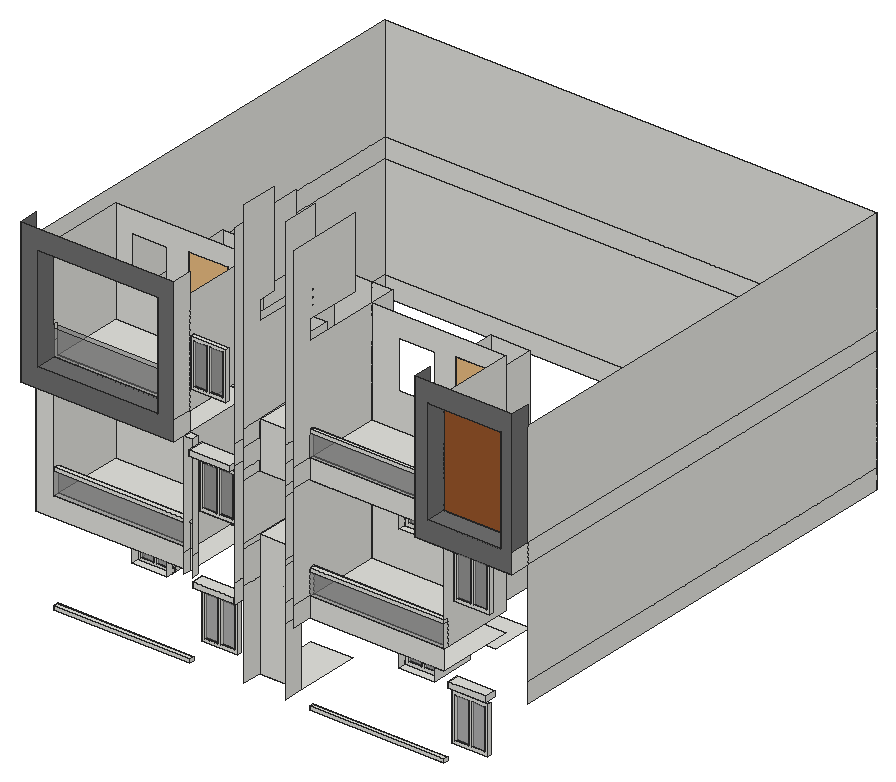
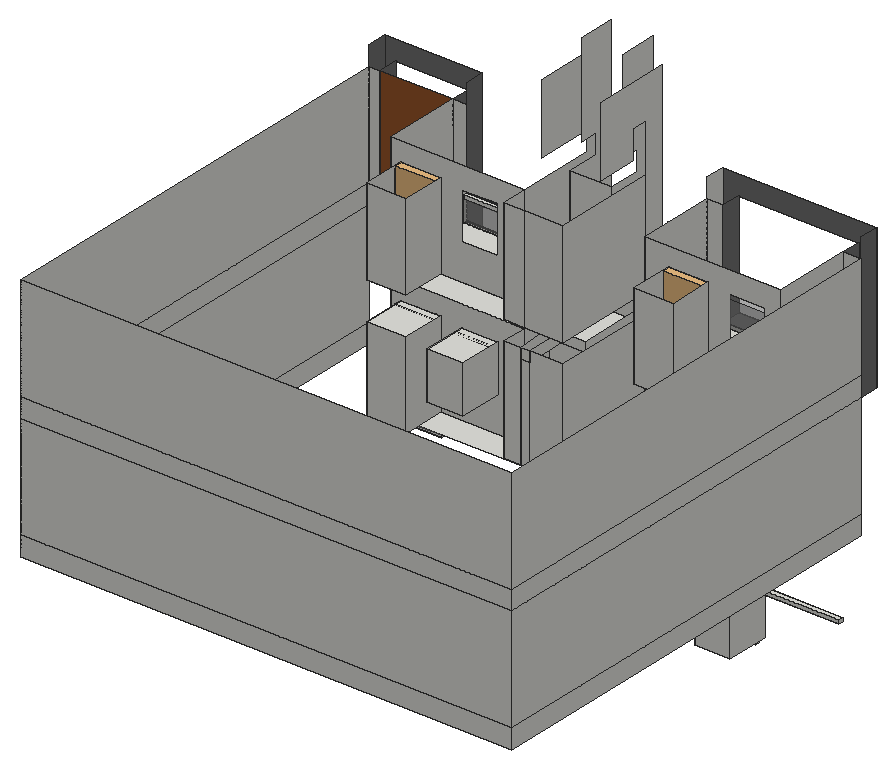
# SketchUp Ruby script. Lengths in inches.
U = 1.inch
M = Sketchup.active_model
def pt(a) = Geom::Point3d.new(a.map { |v| v * U })
def face(e, loops, mat)
  f = e.add_face(loops[0].map { |a| pt(a) })
  loops[1..].each { |l| e.add_face(l.map { |a| pt(a) }).erase! }
  f.material = f.back_material = mat if mat
  f
end
# faces: each face lists its corners as indices into pts; further lists are holes
def faces(e, pts, list, mat = nil) = list.each { |f| face(e, (f[0].is_a?(Array) ? f : [f]).map { |l| l.map { |i| pts[i] } }, mat) }
# xy, xz, yz: faces in a plane at the given z, y or x. An outline is a flat list of corners, or four numbers for a rectangle; further outlines are holes
def ring(l) = l.size == 4 ? [[l[0], l[1]], [l[2], l[1]], [l[2], l[3]], [l[0], l[3]]] : l.each_slice(2).to_a
def flat(e, list, mat, &to3) = list.each { |f| face(e, (f[0].is_a?(Array) ? f : [f]).map { |l| ring(l).map { |u, v| to3.(u, v) } }, mat) }
def xy(e, z, list, mat = nil) = flat(e, list, mat) { |x, y| [x, y, z] }
def xz(e, y, list, mat = nil) = flat(e, list, mat) { |x, z| [x, y, z] }
def yz(e, x, list, mat = nil) = flat(e, list, mat) { |y, z| [x, y, z] }
def lines(e, pts, list) = list.each { |a, b| e.add_line(pt(pts[a]), pt(pts[b])) }
# prism: a flat outline (further loops are holes) pulled along v
def prism(e, loops, v, mat = nil)
  f = face(e, loops, mat); d = Geom::Vector3d.new(v.map { |x| x * U })
  f.pushpull(f.normal.samedirection?(d) ? d.length : -d.length)
end
def box(e, o, s, mat = nil) = prism(e, [[o, [o[0] + s[0], o[1], o[2]], [o[0] + s[0], o[1] + s[1], o[2]], [o[0], o[1] + s[1], o[2]]]], [0, 0, s[2]], mat)
def at(x, y, z, deg = 0) = Geom::Transformation.translation(pt([x, y, z])) * Geom::Transformation.rotation(ORIGIN, Z_AXIS, deg.degrees)
def axes(o, x, y, z) = Geom::Transformation.new([*x, 0, *y, 0, *z, 0, *pt(o).to_a, 1])
def part(name) = M.definitions.add(name)
# library, detail: a bought-in or finely detailed component or shape, given as its bounding box
def library(name, o, s) = part(name).tap { |d| box(d.entities, o, s) }
def detail(e, o, s) = box(e.add_group.entities, o, s)
def put(e, d, t, mat = nil) = e.add_instance(d, t).tap { |i| i.material = mat if mat }
def group(e, t, mat = nil) = e.add_group.tap { |g| g.transformation = t; g.material = mat if mat }.entities
root = M.entities
M.materials.add("Generic").color = [112, 112, 112]
M.materials.add("[Translucent Glass Gray]").color = [128, 128, 128]
M.materials["[Translucent Glass Gray]"].alpha = 0.5
M.materials.add("[Wood Cherry Original]").color = [152, 86, 42]
c1 = part("Group\#2")
xy(c1.entities,0,[[0,0,49,5]])
xy(c1.entities,4.23,[[4.23,0,22.39,2],[26.61,0,44.77,2]])
xy(c1.entities,60.71,[[4.23,0,22.39,2],[26.61,0,44.77,2]])
xy(c1.entities,64.9375,[[0,0,49,5]])
xz(c1.entities,0,[[[0,0,49,64.9375],[26.61,4.23,44.77,60.71],[4.23,4.23,22.39,60.71]]])
xz(c1.entities,2,[[4.23,4.23,22.39,60.71],[26.61,4.23,44.77,60.71]],"[Translucent Glass Gray]")
xz(c1.entities,5,[[0,0,49,64.9375]],"[Translucent Glass Gray]")
yz(c1.entities,0,[[0,0,5,64.9375]])
yz(c1.entities,4.23,[[0,4.23,2,60.71]])
yz(c1.entities,22.39,[[0,4.23,2,60.71]])
yz(c1.entities,26.61,[[0,4.23,2,60.71]])
yz(c1.entities,44.77,[[0,4.23,2,60.71]])
yz(c1.entities,49,[[0,0,5,64.9375]])
c2 = library("Group\#1",[0,0,0],[54.125,10.375,118.625])
box(root,[24,106.875,543.125],[187.17,6.75,4.875])
prism(root,[[[376.97,106.875,543.125],[376.97,112.75,543.125],[547.21,112.75,543.125],[561.52,112.75,543.125],[561.52,106.875,543.125]]],[0,0,4.875])
xy(root,561.83,[[46.11,213.8125,95.11,273.4375],[414.49,213.8125,463.49,273.4375]])
xy(root,563.98,[[307.66,106.875,364.97,195.8125]])
xy(root,626.77,[[46.11,213.8125,95.11,273.4375],[414.49,213.8125,463.49,273.4375]])
xy(root,631.25,[[124.42,213.8125,178.54,273.4375],[492.79,213.8125,546.92,273.4375]])
xy(root,648.74,[[579.7,91.3125,631.39,106.875],[228.07,91.375,285.2,106.875]])
xy(root,656.42,[[579.7,91.3125,631.39,106.875],[228.07,91.375,285.2,106.875]])
xy(root,656.625,[[24,106.875,211.17,213.8125],[376.97,106.875,561.52,213.8125]])
xy(root,683.5,[[24,106.875,211.17,114.3125],[376.97,106.875,561.52,113.625],[376.97,113.625,376.97,213.8125,492.79,213.8125,492.79,273.4375,546.92,273.4375,546.92,213.8125,561.52,213.8125,561.52,113.625],[24,114.3125,24,213.8125,124.42,213.8125,124.42,273.4375,178.54,273.4375,178.54,213.8125,211.17,213.8125,211.17,114.3125]])
xy(root,714,[[24,106.875,211.17,114.3125],[376.97,106.875,561.52,113.625]])
xy(root,718.875,[[24,106.875,211.17,114.3125],[376.97,106.875,561.52,113.625]])
xy(root,732.71,[[46.11,213.8125,95.11,273.4375],[414.49,213.8125,463.49,273.4375]])
xy(root,735.9375,[[307.66,106.875,364.97,195.8125]])
xy(root,797.65,[[46.11,213.8125,95.11,273.4375],[414.49,213.8125,463.49,273.4375]])
xy(root,802.125,[[124.42,213.8125,178.54,273.4375],[492.79,213.8125,546.92,273.4375]])
xy(root,813.67,[[228.07,85,283.64,106.875]])
xy(root,813.8125,[[307.66,106.875,307.66,195.8125,340.97,195.8125,340.97,249.5625,352.97,249.5625,357.49,195.8125,364.97,106.875]])
xy(root,821.36,[[228.07,85,283.64,106.875]])
xy(root,827.5,[[211.17,97.1875,223.17,106.875],[24,106.875,211.17,213.8125],[364.97,106.875,357.49,195.8125,364.97,195.8125],[376.97,106.875,561.52,213.8125]])
xy(root,827.5,[[0,79.8125,211.17,106.875],[542.64,79.8125,676.6875,106.875]],"Generic")
xy(root,854.375,[[189.05,106.875,189.05,114.1875,24,114.1875,24,213.8125,124.42,213.8125,124.42,273.4375,178.54,273.4375,178.54,213.8125,211.17,213.8125,211.17,106.875],[376.97,106.875,542.64,112.0625],[542.64,106.875,542.64,112.0625,376.97,112.0625,376.97,213.8125,492.79,213.8125,492.79,273.4375,546.92,273.4375,546.92,213.8125,561.52,213.8125,561.52,106.875]])
xy(root,854.375,[[24,79.8125,189.05,106.875],[561.52,79.8125,661.8125,106.875]],"Generic")
xy(root,877.8125,[[307.66,106.875,364.97,151]])
xy(root,884.875,[[376.97,106.875,542.64,112.0625]])
xy(root,889.75,[[376.97,106.875,542.64,112.0625]])
xz(root,79.8125,[[[0,827.5,211.17,1025.25],[24,854.375,189.05,998.375]],[[542.64,827.5,676.6875,1025.25],[561.52,854.375,661.8125,998.375]]],"Generic")
xz(root,85,[[228.07,813.67,283.64,821.36]])
xz(root,91.3125,[[579.7,648.74,631.39,656.42]])
xz(root,91.375,[[228.07,648.74,285.2,656.42]])
xz(root,106.875,[[307.66,563.98,364.97,735.9375],[0,656.625,211.17,656.625,211.17,683.5,24,683.5,24,827.5,0,827.5],[376.97,656.625,561.52,683.5],[24,714,211.17,718.875],[376.97,714,561.52,718.875],
  [307.66,813.8125,364.97,877.8125],[0,827.5,211.17,854.375],[376.97,827.5,542.64,854.375],[542.64,827.5,676.6875,854.375],[0,854.375,24,998.375],
  [189.05,854.375,211.17,998.375],[542.64,854.375,561.52,998.375],[661.8125,854.375,676.6875,998.375],[376.97,884.875,542.64,889.75]])
xz(root,106.875,[[24,683.5,211.17,714],[376.97,683.5,561.52,714],[24,854.375,189.05,891],[376.97,854.375,542.64,884.875]],"[Translucent Glass Gray]")
xz(root,106.875,[[561.52,854.375,661.8125,998.375]],"[Wood Cherry Original]")
xz(root,112.0625,[[376.97,884.875,542.64,889.75]])
xz(root,112.0625,[[376.97,854.375,542.64,884.875]],"[Translucent Glass Gray]")
xz(root,113.625,[[376.97,714,561.52,718.875]])
xz(root,113.625,[[376.97,683.5,561.52,714]],"[Translucent Glass Gray]")
xz(root,114.1875,[[24,854.375,189.05,891]],"[Translucent Glass Gray]")
xz(root,114.3125,[[24,714,211.17,718.875]])
xz(root,114.3125,[[24,683.5,211.17,714]],"[Translucent Glass Gray]")
xz(root,151,[[307.66,854.375,347.59,877.8125],[347.59,854.375,364.97,877.8125],[307.66,877.8125,364.97,998.375]])
xz(root,195.8125,[[307.66,683.5,340.97,729],[307.66,729,340.97,735.9375],[340.97,729,357.49,735.9375],[357.49,729,364.97,735.9375],[307.66,735.9375,357.49,735.9375,357.49,827.5,340.97,827.5,340.97,813.8125,307.66,813.8125],
  [307.66,813.8125,340.97,827.5]])
xz(root,213.8125,[[[24,683.5,124.42,683.5,124.42,802.125,178.54,802.125,178.54,683.5,211.17,683.5,211.17,827.5,24,827.5],[46.11,732.71,95.11,797.65]],[[376.97,683.5,492.79,683.5,492.79,802.125,546.92,802.125,546.92,683.5,561.52,683.5,561.52,827.5,376.97,827.5],[414.49,732.71,463.49,797.65]],[[24,854.375,124.42,854.375,124.42,973,178.54,973,178.54,854.375,211.17,854.375,211.17,998.375,24,998.375],[46.11,903.58,95.11,968.52]],[[376.97,854.375,492.79,854.375,492.79,973,546.92,973,546.92,854.375,561.52,854.375,561.52,998.375,376.97,998.375],[414.49,903.58,463.49,968.52]]])
xz(root,249.5625,[[295.66,683.5,340.97,827.5],[340.97,683.5,352.97,813.8125],[352.97,683.5,376.97,827.5],[340.97,813.8125,352.97,827.5],[295.66,854.375,347.59,998.375],
  [347.59,854.375,376.97,998.375]])
xz(root,273.4375,[[46.11,561.83,95.11,626.77],[414.49,561.83,463.49,626.77],[124.42,683.5,178.54,802.125],[492.79,683.5,546.92,802.125],[46.11,732.71,95.11,797.65],
  [414.49,732.71,463.49,797.65],[124.42,854.375,178.54,973],[492.79,854.375,546.92,973]])
xz(root,706.875,[[0,656.625,676.6875,683.5],[0,683.5,676.6875,827.5],[0,827.5,676.6875,854.375],[0,854.375,676.6875,998.375]])
yz(root,0,[[106.875,656.625,706.875,683.5],[106.875,683.5,706.875,827.5],[106.875,827.5,706.875,854.375],[106.875,854.375,706.875,998.375]])
yz(root,0,[[79.8125,827.5,106.875,1025.25]],"Generic")
yz(root,24,[[106.875,683.5,114.3125,714],[114.3125,683.5,213.8125,683.5,213.8125,827.5,106.875,827.5,106.875,718.875,114.3125,718.875],[106.875,714,114.3125,718.875],[114.1875,854.375,213.8125,854.375,213.8125,998.375,106.875,998.375,106.875,895.75,114.1875,895.75]])
yz(root,24,[[79.8125,854.375,106.875,998.375]],"Generic")
yz(root,46.11,[[213.8125,561.83,273.4375,626.77],[213.8125,732.71,273.4375,797.65]])
yz(root,95.11,[[213.8125,561.83,273.4375,626.77],[213.8125,732.71,273.4375,797.65]])
yz(root,124.42,[[213.8125,683.5,273.4375,802.125],[213.8125,854.375,273.4375,973]])
yz(root,178.54,[[213.8125,683.5,273.4375,802.125],[213.8125,854.375,273.4375,973]])
yz(root,189.05,[[106.875,854.375,114.1875,891]])
yz(root,189.05,[[79.8125,854.375,106.875,998.375]],"Generic")
yz(root,211.17,[[97.1875,656.625,106.875,683.5],[97.1875,683.5,97.1875,827.5,213.8125,827.5,213.8125,683.5,114.3125,683.5,114.3125,718.875,106.875,718.875,106.875,683.5],[106.875,683.5,114.3125,714],[106.875,714,114.3125,718.875],[79.8125,827.5,106.875,854.375],
  [79.8125,854.375,106.875,1025.25],[106.875,854.375,213.8125,998.375]])
yz(root,223.17,[[97.1875,656.625,106.875,683.5],[97.1875,683.5,106.875,827.5]])
yz(root,228.07,[[91.375,648.74,106.875,656.42],[85,813.67,106.875,821.36]])
yz(root,283.64,[[85,813.67,106.875,821.36]])
yz(root,285.2,[[91.375,648.74,106.875,656.42]])
yz(root,295.66,[[79.8125,656.625,106.875,683.5],[79.8125,683.5,106.875,827.5],[106.875,683.5,249.5625,827.5],[79.8125,827.5,106.875,854.375],[79.8125,854.375,79.8125,1121.625,184.9375,1121.625,184.9375,1025.25,129.125,1025.25,129.125,1065.0625,106.875,1065.0625,106.875,854.375],
  [106.875,854.375,249.5625,998.375]])
yz(root,307.66,[[79.8125,563.98,106.875,683.5],[79.8125,683.5,106.875,729],[106.875,683.5,195.8125,729],[79.8125,729,106.875,735.9375],[106.875,729,195.8125,735.9375],
  [79.8125,735.9375,195.8125,813.8125],[79.8125,813.8125,106.875,827.5],[106.875,813.8125,195.8125,827.5],[79.8125,827.5,106.875,854.375],[79.8125,854.375,106.875,877.8125],
  [106.875,854.375,151,877.8125],[79.8125,877.8125,151,877.8125,151,998.375,106.875,998.375,106.875,1025.25,130.875,1025.25,130.875,1153.3125,79.8125,1153.3125]])
yz(root,340.97,[[195.8125,813.8125,249.5625,827.5]])
yz(root,364.97,[[79.8125,563.98,106.875,656.625],[79.8125,656.625,106.875,683.5],[79.8125,683.5,106.875,729],[79.8125,729,106.875,735.9375],[106.875,729,195.8125,735.9375],
  [79.8125,735.9375,106.875,813.8125],[106.875,735.9375,195.8125,827.5],[79.8125,813.8125,106.875,827.5],[79.8125,827.5,106.875,854.375],[79.8125,854.375,106.875,877.8125],
  [106.875,854.375,151,877.8125],[79.8125,877.8125,79.8125,1153.3125,130.875,1153.3125,130.875,1025.25,106.875,1025.25,106.875,998.375,151,998.375,151,877.8125]])
yz(root,376.97,[[79.8125,656.625,106.875,683.5],[79.8125,683.5,106.875,683.5,106.875,718.875,113.625,718.875,113.625,683.5,213.8125,683.5,213.8125,827.5,79.8125,827.5],[106.875,683.5,113.625,714],[213.8125,683.5,249.5625,827.5],[106.875,714,113.625,718.875],
  [79.8125,827.5,106.875,854.375],[[79.8125,854.375,106.875,854.375,106.875,889.75,112.0625,889.75,112.0625,854.375,213.8125,854.375,213.8125,998.375,106.875,998.375,106.875,1025.25,184.9375,1025.25,184.9375,1121.625,79.8125,1121.625],[111.28,1057.4,110.76,1057.47,110.28,1057.67,109.86,1057.99,109.55,1058.4,109.35,1058.89,109.28,1059.4,109.35,1059.92,109.55,1060.4,109.86,1060.82,110.28,1061.14,110.76,1061.34,111.28,1061.4,111.79,1061.34,112.28,1061.14,112.69,1060.82,113.01,1060.4,113.21,1059.92,113.28,1059.4,113.21,1058.89,113.01,1058.4,112.69,1057.99,112.28,1057.67,111.79,1057.47],[111.28,1047.72,110.76,1047.78,110.28,1047.98,109.86,1048.3,109.55,1048.72,109.35,1049.2,109.28,1049.72,109.35,1050.23,109.55,1050.72,109.86,1051.13,110.28,1051.45,110.76,1051.65,111.28,1051.72,111.79,1051.65,112.28,1051.45,112.69,1051.13,113.01,1050.72,113.21,1050.23,113.28,1049.72,113.21,1049.2,113.01,1048.72,112.69,1048.3,112.28,1047.98,111.79,1047.78],[111.28,1038.03,110.76,1038.1,110.28,1038.3,109.86,1038.61,109.55,1039.03,109.35,1039.51,109.28,1040.03,109.35,1040.55,109.55,1041.03,109.86,1041.44,110.28,1041.76,110.76,1041.96,111.28,1042.03,111.79,1041.96,112.28,1041.76,112.69,1041.44,113.01,1041.03,113.21,1040.55,113.28,1040.03,113.21,1039.51,113.01,1039.03,112.69,1038.61,112.28,1038.3,111.79,1038.1]],[106.875,854.375,112.0625,884.875],[213.8125,854.375,249.5625,998.375],[106.875,884.875,112.0625,889.75]])
yz(root,414.49,[[213.8125,561.83,273.4375,626.77],[213.8125,732.71,273.4375,797.65]])
yz(root,463.49,[[213.8125,561.83,273.4375,626.77],[213.8125,732.71,273.4375,797.65]])
yz(root,492.79,[[213.8125,683.5,273.4375,802.125],[213.8125,854.375,273.4375,973]])
yz(root,542.64,[[106.875,854.375,112.0625,884.875],[106.875,884.875,112.0625,889.75]])
yz(root,542.64,[[79.8125,827.5,106.875,1025.25]],"Generic")
yz(root,546.92,[[213.8125,683.5,273.4375,802.125],[213.8125,854.375,273.4375,973]])
yz(root,561.52,[[106.875,683.5,113.625,714],[113.625,683.5,113.625,718.875,106.875,718.875,106.875,827.5,213.8125,827.5,213.8125,683.5],[106.875,714,113.625,718.875],[106.875,854.375,213.8125,998.375]])
yz(root,561.52,[[79.8125,854.375,106.875,998.375]],"Generic")
yz(root,579.7,[[91.3125,648.74,106.875,656.42]])
yz(root,631.39,[[91.3125,648.74,106.875,656.42]])
yz(root,661.8125,[[79.8125,854.375,106.875,998.375]],"Generic")
yz(root,676.6875,[[106.875,656.625,706.875,683.5],[106.875,683.5,706.875,827.5],[79.8125,827.5,106.875,854.375],[106.875,827.5,706.875,854.375],[106.875,854.375,706.875,998.375]])
yz(root,676.6875,[[79.8125,854.375,106.875,1025.25]],"Generic")
p = [[364.97,106.875,683.5],[364.97,106.875,729],[364.97,106.875,735.9375],[364.97,106.875,813.8125],[357.49,195.8125,813.8125],[352.97,249.5625,813.8125],
  [352.97,249.5625,683.5],[364.97,106.875,827.5],[357.49,195.8125,827.5],[352.97,249.5625,827.5],[340.97,106.875,683.5],[340.97,195.8125,683.5],
  [340.97,249.5625,683.5],[347.59,151,854.375],[347.59,249.5625,854.375]]
faces(root,p,[[0,1,2,3,4,5,6],[7,8,4,3],[8,9,5,4]])
lines(root,p,[[10,11],[11,12],[13,14]])
put(root,c1,at(46.11,224.0625,560.46))
put(root,c1,at(414.49,224.0625,561.83))
put(root,c1,at(576.76,101.875,575.04))
put(root,c1,at(232.41,101.875,579.98))
put(root,c2,at(492.79,213.8125,683.5))
put(root,c2,at(124.42,213.8125,683.5))
put(root,c1,at(46.11,224.0625,731.33))
put(root,c1,at(414.49,224.0625,732.71))
put(root,c1,at(229.8,101.875,739.91))
put(root,c1,at(579.45,101.875,751.13))
put(root,c2,at(492.79,213.8125,854.375))
put(root,c2,at(124.42,213.8125,854.375))
put(root,c1,at(216.76,101.875,885.58))
